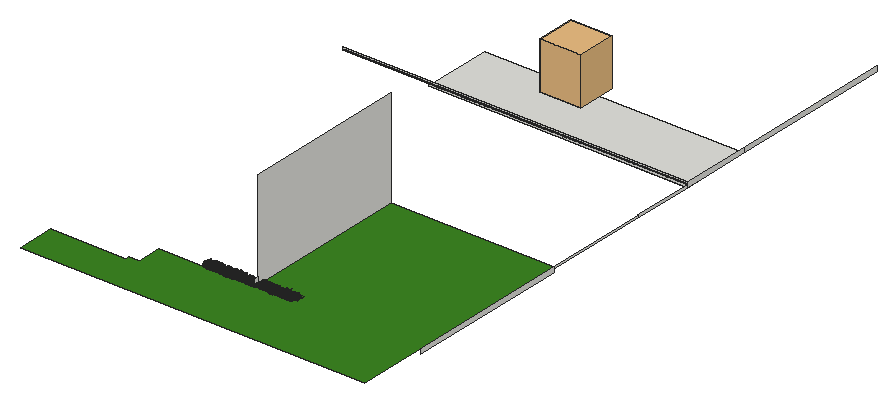
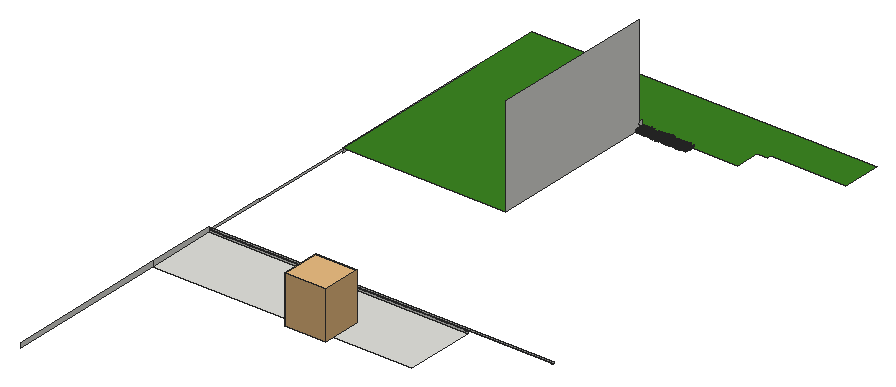
# SketchUp Ruby script. Lengths in inches.
U = 1.inch
M = Sketchup.active_model
def pt(a) = Geom::Point3d.new(a.map { |v| v * U })
def face(e, loops, mat)
  f = e.add_face(loops[0].map { |a| pt(a) })
  loops[1..].each { |l| e.add_face(l.map { |a| pt(a) }).erase! }
  f.material = f.back_material = mat if mat
  f
end
# faces: each face lists its corners as indices into pts; further lists are holes
def faces(e, pts, list, mat = nil) = list.each { |f| face(e, (f[0].is_a?(Array) ? f : [f]).map { |l| l.map { |i| pts[i] } }, mat) }
# xy, xz, yz: faces in a plane at the given z, y or x. An outline is a flat list of corners, or four numbers for a rectangle; further outlines are holes
def ring(l) = l.size == 4 ? [[l[0], l[1]], [l[2], l[1]], [l[2], l[3]], [l[0], l[3]]] : l.each_slice(2).to_a
def flat(e, list, mat, &to3) = list.each { |f| face(e, (f[0].is_a?(Array) ? f : [f]).map { |l| ring(l).map { |u, v| to3.(u, v) } }, mat) }
def xy(e, z, list, mat = nil) = flat(e, list, mat) { |x, y| [x, y, z] }
def xz(e, y, list, mat = nil) = flat(e, list, mat) { |x, z| [x, y, z] }
def yz(e, x, list, mat = nil) = flat(e, list, mat) { |y, z| [x, y, z] }
def lines(e, pts, list) = list.each { |a, b| e.add_line(pt(pts[a]), pt(pts[b])) }
# prism: a flat outline (further loops are holes) pulled along v
def prism(e, loops, v, mat = nil)
  f = face(e, loops, mat); d = Geom::Vector3d.new(v.map { |x| x * U })
  f.pushpull(f.normal.samedirection?(d) ? d.length : -d.length)
end
def box(e, o, s, mat = nil) = prism(e, [[o, [o[0] + s[0], o[1], o[2]], [o[0] + s[0], o[1] + s[1], o[2]], [o[0], o[1] + s[1], o[2]]]], [0, 0, s[2]], mat)
def at(x, y, z, deg = 0) = Geom::Transformation.translation(pt([x, y, z])) * Geom::Transformation.rotation(ORIGIN, Z_AXIS, deg.degrees)
def axes(o, x, y, z) = Geom::Transformation.new([*x, 0, *y, 0, *z, 0, *pt(o).to_a, 1])
def part(name) = M.definitions.add(name)
# library, detail: a bought-in or finely detailed component or shape, given as its bounding box
def library(name, o, s) = part(name).tap { |d| box(d.entities, o, s) }
def detail(e, o, s) = box(e.add_group.entities, o, s)
def put(e, d, t, mat = nil) = e.add_instance(d, t).tap { |i| i.material = mat if mat }
def group(e, t, mat = nil) = e.add_group.tap { |g| g.transformation = t; g.material = mat if mat }.entities
root = M.entities
M.materials.add("Material82").color = [68, 110, 58]
M.materials.add("Material83").color = [48, 90, 38]
M.materials.add("Material84").color = [68, 110, 48]
M.materials.add("Material85").color = [48, 90, 48]
M.materials.add("Material86").color = [58, 110, 58]
M.materials.add("Material87").color = [58, 90, 38]
M.materials.add("Material88").color = [68, 100, 58]
M.materials.add("Material89").color = [48, 100, 38]
M.materials.add("[Color M01]").color = [60, 133, 34]
c1 = part("grass00")
p = [[-0.6875,0.15,0],[-0.56,0.08,5.52],[-0.04,0.03,2.76],[0.48,-0.02,0],[0.35,-0.02,5.52],[-0.1,-0.14,5.52],
  [-0.12,0.65,8.37],[-0.42,0.65,8.37]]
faces(c1.entities,p,[[0,1,2,3],[3,2,4],[1,5,2],[5,4,2],[1,6,5],[4,5,6],[7,6,1]])
c2 = part("Group16\#1")
put(c2.entities,c1,axes([1.44,-0.61,-0.01],[0.05352,0.12609,0],[-0.10704,0.04543,0.07239],[0.06664,-0.02828,0.11628]),"Material85")
put(c2.entities,c1,axes([0.76,-0.15,-0.01],[0.04676,0.24062,0],[-0.23162,0.04501,0.06642],[0.0652,-0.01267,0.23595]),"Material82")
put(c2.entities,c1,axes([0.79,0.01,-0.01],[-0.00606,0.34651,0],[-0.34381,-0.00602,0.0432],[0.04319,0.00076,0.34386]))
put(c2.entities,c1,axes([1,0.23,-0.01],[-0.07192,0.31144,0],[-0.28722,-0.06632,0.1236],[0.12043,0.02781,0.29478]),"Material84")
put(c2.entities,c1,axes([1.66,0.77,-0.01],[-0.13828,0.29651,0],[-0.21551,-0.1005,0.22471],[0.20365,0.09498,0.23779]),"Material89")
put(c2.entities,c1,axes([0.6875,0.52,-0.01],[-0.18126,0.24051,0],[-0.22746,-0.17142,0.09788],[0.07817,0.05891,0.28481]),"Material84")
put(c2.entities,c1,axes([0.68,0.78,-0.01],[-0.215,0.18688,0],[-0.12385,-0.14248,0.21334],[0.13995,0.16101,0.18878]),"Material82")
put(c2.entities,c1,axes([0.56,1,-0.01],[-0.13756,0.07624,0],[-0.06159,-0.11112,0.0927],[0.04494,0.08108,0.12705]),"Material84")
put(c2.entities,c1,axes([0.2,0.64,-0.01],[-0.23729,0.07254,0],[-0.05711,-0.18681,0.153],[0.04473,0.14632,0.19535]),"Material89")
put(c2.entities,c1,axes([0.0625,0.72,-0.01],[-0.28874,0.02525,0],[-0.02179,-0.24916,0.14647],[0.01276,0.14591,0.25012]),"Material82")
put(c2.entities,c1,axes([-0.08,0.62,-0.01],[-0.34089,-0.04187,0],[0.03255,-0.26504,0.216],[-0.02633,0.21439,0.26703]),"Material89")
put(c2.entities,c1,axes([-0.34,0.98,-0.01],[-0.14314,-0.0493,0],[0.04397,-0.12769,0.06843],[-0.02228,0.0647,0.13505]),"Material89")
put(c2.entities,c1,axes([-0.87,1.45,-0.01],[-0.23488,-0.14114,0],[0.13761,-0.22901,0.06087],[-0.03135,0.05217,0.26717]))
put(c2.entities,c1,axes([-0.72,0.77,-0.01],[-0.14208,-0.13251,0],[0.07209,-0.0773,0.16301],[-0.11118,0.11922,0.1057]),"Material89")
put(c2.entities,c1,axes([-0.62,0.43,-0.01],[-0.14845,-0.21203,0],[0.18654,-0.13061,0.12304],[-0.10079,0.07057,0.22772]),"Material82")
put(c2.entities,c1,axes([-0.68,0.29,-0.01],[-0.13639,-0.32136,0],[0.31723,-0.13464,0.05579],[-0.05136,0.0218,0.34462]),"Material83")
put(c2.entities,c1,axes([-0.64,0.125,-0.01],[-0.0458,-0.23569,0],[0.22124,-0.043,0.08276],[-0.08124,0.01579,0.22538]),"Material86")
put(c2.entities,c1,axes([-1.6,-0.03,-0.01],[0.00576,-0.32897,0],[0.27526,0.00482,0.18018],[-0.18015,-0.00315,0.2753]),"Material84")
put(c2.entities,c1,axes([-1.36,-0.31,-0.01],[0.05718,-0.24765,0],[0.18172,0.04196,0.17267],[-0.16825,-0.03885,0.1865]),"Material89")
put(c2.entities,c1,axes([-1.54,-0.72,-0.01],[0.06537,-0.14017,0],[0.13555,0.06321,0.03939],[-0.0357,-0.01665,0.14956]))
put(c2.entities,c1,axes([-1.19,-0.9,-0.01],[0.09597,-0.12735,0],[0.11214,0.08451,0.07557],[-0.06035,-0.04548,0.14042]),"Material88")
put(c2.entities,c1,axes([-0.47,-0.54,-0.01],[0.11588,-0.10072,0],[0.0618,0.0711,0.12124],[-0.07953,-0.0915,0.0942]))
put(c2.entities,c1,axes([-0.47,-0.84,-0.01],[0.11927,-0.0661,0],[0.06603,0.11913,0.00646],[-0.00313,-0.00565,0.13621]),"Material84")
put(c2.entities,c1,axes([-0.38,-1.24,-0.01],[0.28037,-0.08571,0],[0.0618,0.20215,0.20315],[-0.05939,-0.19428,0.21139]),"Material88")
put(c2.entities,c1,axes([-0.06,-0.66,-0.01],[0.22719,-0.01987,0],[0.01247,0.14255,0.17758],[-0.01547,-0.17691,0.1431]),"Material87")
put(c2.entities,c1,axes([0.11,-0.89,-0.01],[0.14882,0.01828,0],[-0.01058,0.08611,0.12229],[0.01491,-0.12138,0.08676]),"Material85")
put(c2.entities,c1,axes([0.25,-0.72,-0.01],[0.20481,0.07053,0],[-0.06206,0.18022,0.10291],[0.03351,-0.0973,0.1906]),"Material85")
put(c2.entities,c1,axes([0.85,-1.42,-0.01],[0.16481,0.09904,0],[-0.09472,0.15762,0.05616],[0.02893,-0.04814,0.18389]),"Material84")
put(c2.entities,c1,axes([1.01,-1.09,-0.01],[0.21858,0.20385,0],[-0.17495,0.1876,0.15339],[0.10462,-0.11218,0.25652]),"Material89")
put(c2.entities,c1,axes([1.01,-0.71,-0.01],[0.08733,0.12473,0],[-0.06445,0.04512,0.13037],[0.1068,-0.07477,0.07867]),"Material85")
c3 = part("Group15\#1")
put(c3.entities,c2,at(0,0,0))
c4 = part("3darcstudiotree_grass00\#1")
put(c4.entities,c3,at(0,0,0))
c5 = library("Flora+17",[-57.52,158.6,-38.64],[66.99,62.88,77.28])
xy(root,-37.75,[[1674.65,932.5,2096.625,1046.93]])
xy(root,-34.17,[[1534.73,273.41,2096.97,273.41,2096.97,659.09,1831.09,659.09,1831.09,381.72,1674.99,381.72,1674.99,341.03,1657.41,341.03,1657.41,335.84,1534.73,335.84]],"[Color M01]")
xz(root,932.5,[[1674.65,-37.75,2096.625,-37.75,2096.625,-34.17,1896.9375,-34.17,1896.9375,-34.6875,1674.65,-34.6875],[1674.65,-34.6875,1896.9375,-34.17],[1674.65,-34.17,2096.625,-33.75],[1534.38,-33.42,2096.625,-32.8],[1534.38,-32.8,2096.625,-29.74]])
yz(root,1831.09,[[381.72,-34.17,387.84,-22.8],[387.84,-34.17,659.09,126.75]])
yz(root,2096.625,[[660.69,-37.75,831.37,-34.75],[831.37,-37.75,932.5,-34.17],[932.5,-37.75,1046.93,-29.74],[1046.93,-37.75,1318.18,-29.74]])
yz(root,2096.97,[[387.84,-42.1875,659.09,-34.17]])
put(root,c4,axes([1778.76,381.9375,-34.17],[4.09331,0.01199,0],[-0.0289,1.53398,-0.04293],[-0.00148,0.07869,1.35522]))
put(root,c4,axes([1826.625,381.87,-34.17],[-3.29126,-0.79109,0],[1.80045,-1.16502,-0.03312],[0.11366,-0.07354,1.70984]))
put(root,c4,axes([1789.76,381.79,-34.17],[1.86032,1.34861,0],[-2.96544,0.63621,-0.01685],[-0.11323,0.02429,1.93576]))
put(root,c4,axes([1785.04,381.58,-34.17],[-4.56188,0.50767,0],[-1.2186,-1.7031,-0.00145],[-0.00214,-0.00299,1.8291]))
put(root,c4,axes([1755.57,382.11,-34.17],[-1.58728,-1.19948,0],[3.58979,-0.73882,-0.00435],[0.01908,-0.00393,1.50222]))
put(root,c4,axes([1768.33,382,-34.17],[-3.20908,-0.65771,0],[1.52004,-1.1535,-0.02241],[0.0705,-0.0535,1.68548]))
put(root,c4,axes([1859.54,381.91,-34.17],[0.845,1.5364,0],[-3.22221,0.27563,-0.00976],[-0.06274,0.00537,1.62508]))
put(root,c4,axes([1797.79,382.19,-34.17],[-3.10229,-1.16988,0],[2.93363,-1.20992,-0.00934],[0.03186,-0.01314,1.57129]))
put(root,c4,axes([1884.03,382.97,-34.17],[3.21747,0.34612,0],[-1.00705,1.45598,-0.00322],[-0.00588,0.0085,1.99197]))
put(root,c4,axes([1855.76,383.26,-34.17],[2.05313,-1.14667,0],[3.04328,0.84748,-0.00946],[0.04471,0.01245,1.61646]))
put(root,c4,axes([1759.2,382.88,-34.17],[1.49785,1.29889,0],[-3.32043,0.59552,-0.00419],[-0.02419,0.00434,1.73548]))
put(root,c4,axes([1876.59,383.19,-34.17],[-2.06721,-1.47479,0],[2.97534,-0.64864,-0.04183],[0.21369,-0.04658,1.48723]))
put(root,c4,axes([1804.75,383.36,-34.17],[3.7963,-0.32727,0],[0.82791,1.49367,-0.02018],[0.02229,0.04022,1.50307]))
put(root,c4,axes([1814.8125,383.2,-34.17],[3.44974,0.13102,0],[-0.35474,1.45265,-0.03978],[-0.02715,0.11118,1.9745]))
put(root,c4,axes([1862.49,383.25,-34.17],[3.55632,0.05998,0],[-0.17821,1.64336,-0.05798],[-0.01271,0.11725,1.60438]))
put(root,c4,axes([1886.81,382.91,-34.17],[-3.26011,-0.21751,0],[0.57833,-1.34815,-0.02254],[0.02017,-0.04702,1.39425]))
put(root,c4,axes([1822.11,383.16,-34.17],[-2.04014,-1.04561,0],[3.14641,-0.95481,-0.03027],[0.11908,-0.03613,1.47708]))
put(root,c4,axes([1798.47,382.96,-34.17],[-4.12072,-0.27119,0],[0.6549,-1.54771,-0.03361],[0.02858,-0.06755,1.54092]))
put(root,c4,axes([1756.15,383.13,-34.17],[-3.19208,-0.59663,0],[1.68588,-1.40285,-0.03887],[0.08271,-0.06882,1.46596]))
put(root,c4,axes([1765.42,383.21,-34.17],[-3.36658,1.12781,0],[-2.16506,-1.00516,-0.00331],[-0.01262,-0.00586,1.47415]))
put(root,c4,axes([1772.27,383.34,-34.17],[-3.68407,-0.02356,0],[0.06081,-1.47897,-0.00434],[0.00034,-0.00838,1.37632]))
put(root,c4,axes([1843.85,384.11,-34.17],[3.71353,-0.51552,0],[1.56304,1.75115,-0.03514],[0.05159,0.0578,1.55988]))
put(root,c4,axes([1795.67,383.45,-34.17],[0.6827,1.82438,0],[-3.27697,0.19072,-0.00575],[-0.03023,0.00176,1.31904]))
put(root,c4,axes([1789.77,383.66,-34.17],[2.40726,1.00896,0],[-2.45133,0.90962,-0.04643],[-0.23456,0.08704,1.7498]))
put(root,c4,axes([1782.6875,384.03,-34.17],[0.00434,-1.45328,0],[3.77222,0.00175,-0.01884],[0.09694,0.00004,1.45492]))
put(root,c4,axes([1865.57,384.18,-34.17],[1.06558,-1.7102,0],[3.88793,0.37676,-0.05295],[0.33853,0.03281,1.97565]))
put(root,c4,axes([1811.59,383.8,-34.17],[-4.10821,-0.63147,0],[1.40621,-1.42285,-0.03755],[0.0732,-0.07407,1.55797]))
put(root,c4,axes([1827.38,384.18,-34.17],[3.5779,0.22372,0],[-0.65952,1.64048,-0.02805],[-0.02776,0.06904,1.99488]))
put(root,c4,axes([1838.32,384.14,-34.17],[-0.99859,-1.42329,0],[3.17499,-0.34645,-0.0133],[0.07574,-0.00827,1.45899]))
put(root,c4,axes([1833.61,383.61,-34.17],[-2.82382,0.83563,0],[-2.68315,-1.4102,-0.02868],[-0.0714,-0.03753,1.39]))
put(root,c4,axes([1872.5,383.98,-34.17],[-4.01729,-0.17274,0],[0.40562,-1.46709,-0.05296],[0.03317,-0.11998,1.62079]))
put(root,c4,axes([1777.8,383.9,-34.17],[-4.10797,-0.04724,0],[0.09871,-1.33508,-0.0193],[0.00442,-0.0598,1.99558]))
put(root,c4,axes([1849.37,384.04,-34.17],[-1.96777,1.0795,0],[-3.29786,-0.93497,-0.0015],[-0.00541,-0.00153,1.35234]))
put(root,c4,axes([1816.79,385.02,-34.17],[0.94515,-1.66762,0],[4.07339,0.35906,-0.0396],[0.18346,0.01617,1.48525]))
put(root,c4,axes([1866.6875,385.11,-34.17],[3.84561,-0.02617,0],[0.07345,1.67847,-0.0287],[0.00308,0.07036,1.98369]))
put(root,c4,axes([1843.18,385.32,-34.17],[1.96372,-1.5045,0],[4.10696,0.83372,-0.06088],[0.26019,0.05282,1.6642]))
put(root,c4,axes([1856.04,385.28,-34.17],[3.54187,-0.26159,0],[0.80325,1.69151,-0.05648],[0.04449,0.09368,1.39957]))
put(root,c4,axes([1826.3125,385.49,-34.17],[0.99321,-1.58581,0],[3.96504,0.38623,-0.04714],[0.20087,0.01957,1.34372]))
put(root,c4,axes([1811.89,385.62,-34.17],[-0.45128,-1.33361,0],[4.22591,-0.22241,-0.03174],[0.17504,-0.00921,1.77768]))
put(root,c4,axes([1793.8,385.82,-34.17],[3.22644,-0.51746,0],[1.32565,1.28555,-0.02601],[0.05462,0.05297,1.4702]))
put(root,c4,axes([1773.51,385.76,-34.17],[3.6798,1.00569,0],[-2.52504,1.43694,-0.01195],[-0.02817,0.01603,1.37528]))
put(root,c4,axes([1838.12,385.57,-34.17],[1.82247,1.66574,0],[-4.14446,0.70523,-0.02206],[-0.09849,0.01676,1.64521]))
put(root,c4,axes([1797.98,385.65,-34.17],[-2.84959,-0.68183,0],[2.166,-1.40791,-0.04577],[0.14869,-0.09665,1.96036]))
put(root,c4,axes([1820.01,385.93,-34.17],[4.19345,0.64908,0],[-1.43857,1.4455,-0.00074],[-0.00143,0.00144,1.56313]))
put(root,c4,axes([1861.98,385.29,-34.17],[-3.99369,0.93834,0],[-2.11578,-1.40055,-0.00882],[-0.02078,-0.01375,1.42641]))
put(root,c4,axes([1875.87,385.48,-34.17],[-3.34892,0.63546,0],[-1.79553,-1.4717,-0.05656],[-0.12201,-0.10001,1.54444]))
put(root,c4,axes([1805.91,386.15,-34.17],[2.39093,-1.03283,0],[3.02488,1.08907,-0.05494],[0.24262,0.08735,1.83588]))
put(root,c4,axes([1872.07,385.55,-34.17],[-2.29973,1.37871,0],[-3.78776,-0.98265,-0.04701],[-0.18775,-0.04871,1.62457]))
put(root,c4,axes([1765.36,385.77,-34.17],[0.30119,1.56993,0],[-3.74927,0.11187,-0.04286],[-0.21599,0.00644,1.42447]))
put(root,c4,axes([1886.25,386.3,-34.17],[4.21864,0.55626,0],[-1.1609,1.36932,-0.01696],[-0.03551,0.04188,1.81122]))
put(root,c4,axes([1782.67,385.875,-34.17],[-3.66261,0.69653,0],[-1.57298,-1.28643,-0.02015],[-0.06083,-0.04975,1.88684]))
put(root,c4,axes([1849.93,385.9,-34.17],[-0.80631,1.56039,0],[-4.1673,-0.33492,-0.00834],[-0.04436,-0.00356,1.72954]))
put(root,c4,axes([1753.72,386.3,-34.17],[-0.23965,1.40351,0],[-3.9598,-0.10516,-0.04305],[-0.25813,-0.00685,1.78778]))
put(root,c4,axes([1779.58,386.33,-34.17],[-0.04316,1.58062,0],[-4.72981,-0.02009,-0.05791],[-0.26281,-0.00112,1.60897]))
put(root,c4,axes([1882.11,386.28,-34.17],[-3.37719,0.09425,0],[-0.3007,-1.67585,-0.01026],[-0.00386,-0.0215,1.70108]))
put(root,c4,axes([1787.01,386.49,-34.17],[0.64791,1.78613,0],[-4.32576,0.24405,-0.02596],[-0.10407,0.00587,1.32635]))
put(root,c4,axes([1760.69,386.58,-34.17],[-3.52632,-0.01876,0],[0.05142,-1.50323,-0.03579],[0.00272,-0.07942,1.60809]))
put(root,c4,axes([1834.4,386.45,-34.17],[-1.94441,1.40342,0],[-3.94861,-0.85085,-0.04785],[-0.22127,-0.04768,1.77706]))
put(root,c4,axes([1777.84,387.22,-34.17],[0.58086,-1.47611,0],[3.37891,0.2068,-0.00401],[0.02817,0.00172,1.82024]))
put(root,c4,axes([1883.01,387.4375,-34.17],[3.52188,-1.04915,0],[2.07703,1.0844,-0.01203],[0.05383,0.0281,1.91781]))
put(root,c4,axes([1806.66,387.51,-34.17],[-0.2827,-1.72948,0],[4.63241,-0.11777,-0.03565],[0.15653,-0.00398,1.53082]))
put(root,c4,axes([1773.74,387.43,-34.17],[-3.67064,-0.9709,0],[1.88491,-1.10833,-0.03319],[0.11926,-0.07012,1.63594]))
put(root,c4,axes([1766.1875,387.83,-34.17],[3.50639,-1.07574,0],[2.8139,1.42651,-0.05588],[0.16686,0.08459,1.67045]))
put(root,c4,axes([1860.8,387.78,-34.17],[1.01558,-1.39222,0],[4.1939,0.47581,-0.0144],[0.07646,0.00867,1.80693]))
put(root,c4,axes([1821.69,387.48,-34.17],[3.41924,1.14131,0],[-2.67356,1.24575,-0.04954],[-0.1842,0.08583,1.78537]))
put(root,c4,axes([1848.24,387.26,-34.17],[0.28845,1.63387,0],[-3.6901,0.10132,-0.01352],[-0.07291,0.002,1.49862]))
put(root,c4,axes([1759.57,387.49,-34.17],[2.65644,1.45338,0],[-3.09672,0.88031,-0.01552],[-0.06337,0.01801,1.43977]))
put(root,c4,axes([1831,387.98,-34.17],[1.87129,-1.65871,0],[3.35394,0.58849,-0.03607],[0.16948,0.02974,1.41495]))
put(root,c4,axes([1886.6875,387.96,-34.17],[3.01548,-1.43579,0],[2.66285,0.86981,-0.04892],[0.23141,0.07559,1.59182]))
put(root,c4,axes([1794.03,387.43,-34.17],[-3.80321,-0.44648,0],[1.10938,-1.46975,-0.0137],[0.0187,-0.02478,1.39479]))
put(root,c4,axes([1878,387.32,-34.17],[-3.21998,0.77713,0],[-2.13854,-1.37813,-0.04749],[-0.1058,-0.06818,1.3106]))
put(root,c4,axes([1870.43,388.125,-34.17],[4.18213,-0.23196,0],[0.63555,1.78214,-0.01318],[0.01066,0.02989,1.98636]))
put(root,c4,axes([1812.02,388.09,-34.17],[-2.48368,-1.57939,0],[3.38438,-0.82775,-0.05324],[0.27998,-0.06848,1.84703]))
put(root,c4,axes([1843.01,388.25,-34.17],[4.18444,0.27637,0],[-0.72897,1.71663,-0.00046],[-0.00033,0.00077,1.40239]))
put(root,c4,axes([1855.5,388.3,-34.17],[3.48402,0.19943,0],[-0.6366,1.72969,-0.0224],[-0.01372,0.03729,1.41716]))
put(root,c4,axes([1840.22,388.375,-34.17],[2.76674,0.9412,0],[-2.67302,1.22208,-0.02494],[-0.08686,0.03971,1.63549]))
put(root,c4,axes([1787.53,388.16,-34.17],[2.43664,1.45627,0],[-2.82206,0.73439,-0.04277],[-0.22349,0.05816,1.58679]))
put(root,c4,axes([1867.12,388.69,-34.17],[1.32588,-1.61709,0],[3.49004,0.44505,-0.02554],[0.12415,0.01583,1.40467]))
put(root,c4,axes([1828.17,388.49,-34.17],[3.90165,0.71674,0],[-1.5443,1.30747,-0.0112],[-0.02712,0.02296,1.5714]))
put(root,c4,axes([1753.34,388.16,-34.17],[-0.87127,1.65753,0],[-3.69619,-0.30217,-0.02464],[-0.15319,-0.01252,1.79662]))
put(root,c4,axes([1814.67,388.28,-34.17],[-2.56197,0.85481,0],[-2.91428,-1.35846,-0.04396],[-0.15305,-0.07134,1.82298]))
put(root,c4,axes([1783.93,388.47,-34.17],[-0.0946,1.80399,0],[-4.6355,-0.03781,-0.04199],[-0.20347,-0.00166,1.68448]))
put(root,c4,axes([1800.6,388.59,-34.17],[-3.95195,-0.11479,0],[0.31612,-1.69258,-0.00991],[0.00383,-0.02049,1.69565]))
put(root,c4,axes([1839.74,389.54,-34.17],[2.92757,-1.05075,0],[2.58194,1.11883,-0.00947],[0.03015,0.01306,1.36019]))
put(root,c4,axes([1782.8125,389.5625,-34.17],[4.14299,-0.56741,0],[1.47163,1.6712,-0.03586],[0.0631,0.07166,1.80381]))
put(root,c4,axes([1861.95,389.64,-34.17],[2.43403,-1.47369,0],[3.95187,1.01516,-0.04483],[0.17665,0.04538,1.66248]))
put(root,c4,axes([1789.87,389.7,-34.17],[2.20641,-0.98098,0],[3.35125,1.17232,-0.037],[0.12603,0.04409,1.52862]))
put(root,c4,axes([1848.38,389.625,-34.17],[-0.61871,-1.33799,0],[4.52735,-0.32561,-0.01194],[0.05418,-0.0039,1.59034]))
put(root,c4,axes([1814.74,389.36,-34.17],[-3.07207,1.32257,0],[-2.98229,-1.07739,-0.02313],[-0.10886,-0.03933,1.93523]))
put(root,c4,axes([1873.13,389.9,-34.17],[-2.58829,-1.32174,0],[3.13096,-0.95358,-0.00917],[0.03927,-0.01196,1.60374]))
put(root,c4,axes([1806.86,389.68,-34.17],[1.17272,1.70605,0],[-3.75992,0.40197,-0.02312],[-0.1149,0.01228,1.50331]))
put(root,c4,axes([1884.65,389.68,-34.17],[0.77928,1.7442,0],[-4.29167,0.29822,-0.04576],[-0.22745,0.0158,1.64855]))
put(root,c4,axes([1776.29,390.06,-34.17],[-3.05504,-0.78096,0],[2.06441,-1.25601,-0.04254],[0.14556,-0.08856,1.78955]))
put(root,c4,axes([1855.02,389.87,-34.17],[-0.96871,1.48497,0],[-4.54289,-0.46091,-0.03008],[-0.14643,-0.01486,1.76703]))
put(root,c4,axes([1754.1875,389.98,-34.17],[0.67536,1.71011,0],[-3.33591,0.2049,-0.00889],[-0.04851,0.00298,1.39664]))
put(root,c4,axes([1825.91,390.38,-34.17],[2.90547,0.96842,0],[-2.50521,1.16898,-0.00305],[-0.01073,0.00501,1.58836]))
put(root,c4,axes([1800.18,390.13,-34.17],[-4.49885,0.1512,0],[-0.3136,-1.45126,-0.04489],[-0.02566,-0.11876,1.86365]))
put(root,c4,axes([1823.8,390.39,-34.17],[-2.30012,-1.16982,0],[2.63485,-0.80575,-0.0081],[0.04804,-0.01469,1.87526]))
put(root,c4,axes([1843.83,390.18,-34.17],[-3.42471,-0.0278,0],[0.09598,-1.83904,-0.05231],[0.00587,-0.11256,1.90792]))
put(root,c4,axes([1833.19,390.48,-34.17],[-1.92512,-1.14787,0],[3.14134,-0.81939,-0.00554],[0.02611,-0.00681,1.59445]))
put(root,c4,axes([1766.73,390.12,-34.17],[-1.98309,1.36521,0],[-3.29696,-0.74485,-0.00674],[-0.03007,-0.00679,1.46389]))
put(root,c4,axes([1875.54,390.5,-34.17],[2.80131,1.49669,0],[-2.81369,0.81906,-0.03251],[-0.16371,0.04766,1.64081]))
put(root,c4,axes([1809.58,390.83,-34.17],[3.47876,0.69717,0],[-2.07434,1.60981,-0.02666],[-0.05222,0.04053,1.48409]))
put(root,c4,axes([1772.64,390.43,-34.17],[-2.752,0.72492,0],[-2.08218,-1.22939,-0.04884],[-0.13401,-0.07912,1.38796]))
put(root,c4,axes([1762.62,390.3,-34.17],[-2.99935,1.42497,0],[-3.08029,-1.00838,-0.00469],[-0.01919,-0.00628,1.59556]))
put(root,c4,axes([1793.5625,390.95,-34.17],[-4.04158,-0.94067,0],[1.75814,-1.17484,-0.01139],[0.03404,-0.02275,1.52439]))
put(root,c4,axes([1866.41,390.95,-34.17],[-2.36734,0.93793,0],[-2.35302,-0.92369,-0.04592],[-0.18701,-0.07341,1.42994]))
put(root,c4,axes([1825.42,391.58,-34.17],[3.51961,1.01739,0],[-2.56437,1.37974,-0.04132],[-0.14142,0.07609,1.88254]))
put(root,c4,axes([1767.57,391.75,-34.17],[-0.91614,-1.55858,0],[4.47177,-0.40881,-0.01344],[0.0544,-0.00497,1.42931]))
put(root,c4,axes([1797.95,391.89,-34.17],[3.44355,0.26807,0],[-0.70938,1.41724,-0.02055],[-0.0272,0.05435,1.87683]))
put(root,c4,axes([1795.01,392.14,-34.17],[4.25801,-0.4781,0],[1.08249,1.49942,-0.0361],[0.05003,0.0693,1.4995]))
put(root,c4,axes([1850.33,391.64,-34.17],[-4.54557,-0.49368,0],[1.16722,-1.67149,-0.00177],[0.00248,-0.00355,1.73275]))
put(root,c4,axes([1789.41,391.57,-34.17],[-3.5428,1.01388,0],[-2.21614,-1.2044,-0.01293],[-0.05166,-0.02807,1.92389]))
put(root,c4,axes([1770.96,392.21,-34.17],[3.58378,0.39823,0],[-1.22974,1.72119,-0.04858],[-0.06101,0.08539,1.57379]))
put(root,c4,axes([1812.75,391.72,-34.17],[-3.51929,1.02852,0],[-2.47816,-1.3188,-0.03727],[-0.13373,-0.07117,1.88005]))
put(root,c4,axes([1866.02,392.18,-34.17],[2.58784,1.12355,0],[-2.76399,0.99014,-0.01914],[-0.07187,0.02574,1.41957]))
put(root,c4,axes([1754.97,392.6,-34.17],[2.58879,-1.26718,0],[2.80569,0.89147,-0.02709],[0.14156,0.04498,1.8123]))
put(root,c4,axes([1881,392.74,-34.17],[3.2252,-1.24507,0],[3.05222,1.22967,-0.00616],[0.02183,0.0088,1.65812]))
put(root,c4,axes([1839.43,392,-34.17],[-3.2702,-0.26148,0],[0.88726,-1.72581,-0.02938],[0.02304,-0.04482,1.3208]))
put(root,c4,axes([1777.58,392.63,-34.17],[0.31357,-1.68647,0],[3.44554,0.09964,-0.00239],[0.01314,0.00038,1.42634]))
put(root,c4,axes([1833.91,392.63,-34.17],[3.46613,-0.34597,0],[1.04996,1.63602,-0.03471],[0.05136,0.08002,1.93398]))
put(root,c4,axes([1804.82,392.28,-34.17],[-3.51186,-0.721,0],[1.80955,-1.37083,-0.02288],[0.05511,-0.04175,1.53217]))
put(root,c4,axes([1887.34,392.1,-34.17],[-1.83571,1.27258,0],[-3.25848,-0.73105,-0.04597],[-0.18825,-0.04223,1.32398]))
put(root,c4,axes([1873.0625,392.78,-34.17],[3.30404,-0.44467,0],[1.11823,1.29225,-0.02189],[0.05068,0.05857,1.86062]))
put(root,c4,axes([1858.64,392.7,-34.17],[3.79709,-0.21086,0],[0.51761,1.44966,-0.04526],[0.04066,0.11387,1.7925]))
put(root,c4,axes([1780.98,392.78,-34.17],[4.65922,-0.05932,0],[0.11762,1.43686,-0.01793],[0.0038,0.04639,1.79317]))
put(root,c4,axes([1817.22,392.66,-34.17],[-2.71598,-1.39793,0],[3.51357,-1.0617,-0.04805],[0.18587,-0.05616,1.61679]))
put(root,c4,axes([1853.75,392.33,-34.17],[-1.13728,1.56272,0],[-3.25789,-0.36875,-0.04255],[-0.28342,-0.03208,1.76068]))
put(root,c4,axes([1842.53,393.07,-34.17],[3.34396,-0.78628,0],[2.01461,1.33256,-0.01626],[0.05098,0.03372,1.80561]))
put(root,c4,axes([1876.06,392.48,-34.17],[-3.32221,0.63503,0],[-1.46009,-1.18802,-0.04774],[-0.13797,-0.11226,1.66266]))
put(root,c4,axes([1823.3,392.63,-34.17],[-4.26955,0.05297,0],[-0.11438,-1.43394,-0.03177],[-0.00727,-0.09116,1.98473]))
put(root,c4,axes([1760.34,393.07,-34.17],[-3.0378,0.91986,0],[-2.50548,-1.28689,-0.05552],[-0.17911,-0.092,1.63365]))
put(root,c4,axes([1761.27,393.82,-34.17],[2.17543,-1.37172,0],[2.92508,0.72149,-0.0272],[0.16226,0.04002,1.81972]))
put(root,c4,axes([1838.23,393.8,-34.17],[1.37568,-1.20584,0],[3.91752,0.6951,-0.04402],[0.22671,0.04023,1.81837]))
put(root,c4,axes([1860.46,393.71,-34.17],[3.59871,0.46514,0],[-1.32691,1.59666,-0.04711],[-0.07156,0.0861,1.55738]))
put(root,c4,axes([1848.22,393.91,-34.17],[-2.0544,-1.27697,0],[2.98947,-0.74801,-0.00968],[0.05342,-0.01337,1.73508]))
put(root,c4,axes([1783.73,393.93,-34.17],[-1.59587,-1.14266,0],[4.12201,-0.89537,-0.06742],[0.26463,-0.05748,1.58058]))
put(root,c4,axes([1887.16,394.33,-34.17],[3.62221,-0.68496,0],[1.51778,1.24833,-0.03326],[0.08982,0.07387,1.64345]))
put(root,c4,axes([1878.4,393.89,-34.17],[-0.69326,1.7064,0],[-4.31448,-0.27262,-0.01053],[-0.04979,-0.00315,1.56894]))
put(root,c4,axes([1873.7,394.22,-34.17],[2.26243,1.54744,0],[-3.43917,0.78203,-0.02249],[-0.10645,0.02421,1.62577]))
put(root,c4,axes([1798.44,394.22,-34.17],[0.25287,1.52902,0],[-3.62555,0.09325,-0.03468],[-0.21891,0.00563,1.72254]))
put(root,c5,at(1855.89,846.28,4.4375))
